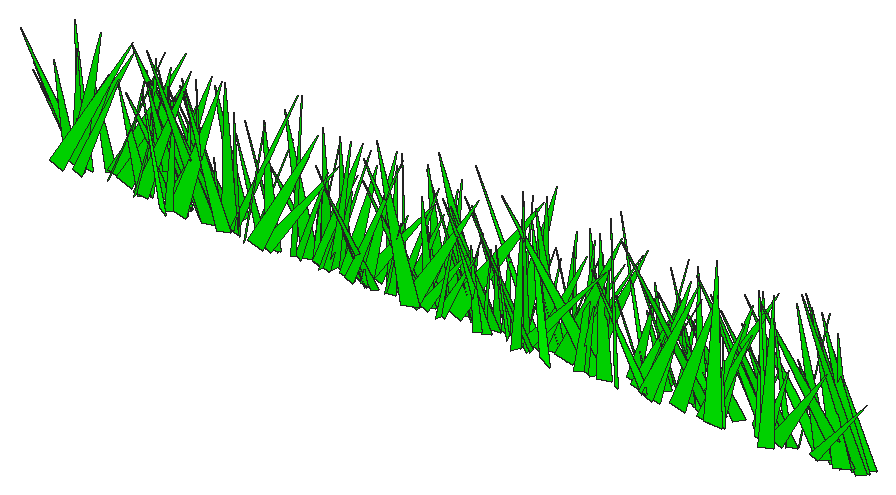
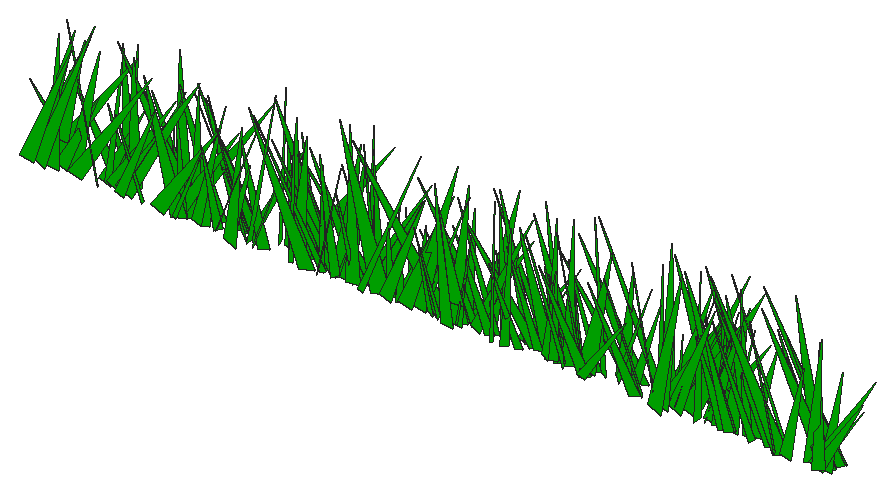
# SketchUp Ruby script. Lengths in inches.
U = 1.inch
M = Sketchup.active_model
def pt(a) = Geom::Point3d.new(a.map { |v| v * U })
def face(e, loops, mat)
  f = e.add_face(loops[0].map { |a| pt(a) })
  loops[1..].each { |l| e.add_face(l.map { |a| pt(a) }).erase! }
  f.material = f.back_material = mat if mat
  f
end
# faces: each face lists its corners as indices into pts; further lists are holes
def faces(e, pts, list, mat = nil) = list.each { |f| face(e, (f[0].is_a?(Array) ? f : [f]).map { |l| l.map { |i| pts[i] } }, mat) }
# xy, xz, yz: faces in a plane at the given z, y or x. An outline is a flat list of corners, or four numbers for a rectangle; further outlines are holes
def ring(l) = l.size == 4 ? [[l[0], l[1]], [l[2], l[1]], [l[2], l[3]], [l[0], l[3]]] : l.each_slice(2).to_a
def flat(e, list, mat, &to3) = list.each { |f| face(e, (f[0].is_a?(Array) ? f : [f]).map { |l| ring(l).map { |u, v| to3.(u, v) } }, mat) }
def xy(e, z, list, mat = nil) = flat(e, list, mat) { |x, y| [x, y, z] }
def xz(e, y, list, mat = nil) = flat(e, list, mat) { |x, z| [x, y, z] }
def yz(e, x, list, mat = nil) = flat(e, list, mat) { |y, z| [x, y, z] }
def lines(e, pts, list) = list.each { |a, b| e.add_line(pt(pts[a]), pt(pts[b])) }
# prism: a flat outline (further loops are holes) pulled along v
def prism(e, loops, v, mat = nil)
  f = face(e, loops, mat); d = Geom::Vector3d.new(v.map { |x| x * U })
  f.pushpull(f.normal.samedirection?(d) ? d.length : -d.length)
end
def box(e, o, s, mat = nil) = prism(e, [[o, [o[0] + s[0], o[1], o[2]], [o[0] + s[0], o[1] + s[1], o[2]], [o[0], o[1] + s[1], o[2]]]], [0, 0, s[2]], mat)
def at(x, y, z, deg = 0) = Geom::Transformation.translation(pt([x, y, z])) * Geom::Transformation.rotation(ORIGIN, Z_AXIS, deg.degrees)
def axes(o, x, y, z) = Geom::Transformation.new([*x, 0, *y, 0, *z, 0, *pt(o).to_a, 1])
def part(name) = M.definitions.add(name)
# library, detail: a bought-in or finely detailed component or shape, given as its bounding box
def library(name, o, s) = part(name).tap { |d| box(d.entities, o, s) }
def detail(e, o, s) = box(e.add_group.entities, o, s)
def put(e, d, t, mat = nil) = e.add_instance(d, t).tap { |i| i.material = mat if mat }
def group(e, t, mat = nil) = e.add_group.tap { |g| g.transformation = t; g.material = mat if mat }.entities
root = M.entities
M.materials.add("[0065_Lime]").color = [0, 255, 0]
c1 = part("fur_instance\#9")
p = [[0.8125,0,1.79],[0.67,-0.02,1.48],[0,-0.11,0],[0,0.11,0]]
faces(c1.entities,p,[[0,1,2,3]])
put(root,c1,axes([44.13,30.08,1.48],[-0.34451,1.18305,1.71198],[-8.4647,0.01946,-1.57758],[-1.91364,-0.29905,6.67002]),"[0065_Lime]")
put(root,c1,axes([64.73,30.03,1.48],[-8.65936,0.15726,2.6065],[-0.41279,-1.27348,1.6673],[3.36902,0.24818,6.90374]),"[0065_Lime]")
put(root,c1,axes([19.73,29.78,1.48],[-6.79777,0.33019,0.23005],[-1.91703,-0.83902,2.87402],[1.38808,0.4583,5.09585]),"[0065_Lime]")
put(root,c1,axes([61.13,30.51,1.48],[-1.56517,-0.52919,0.70817],[3.60677,-0.24741,-0.92094],[1.39004,0.0461,3.18697]),"[0065_Lime]")
put(root,c1,axes([37.86,30.3,1.48],[6.89513,0.62378,0.88009],[-4.56524,0.95182,1.05921],[-0.18718,-0.23644,6.58578]),"[0065_Lime]")
put(root,c1,axes([28.67,30.09,1.48],[2.67792,1.06969,0.54376],[-7.35877,0.33413,1.95261],[2.06045,-0.19692,6.26692]),"[0065_Lime]")
put(root,c1,axes([27.64,30.03,1.48],[6.77204,0.25909,1.43448],[-1.29307,0.95444,-1.73753],[-2.19947,0.23661,5.43816]),"[0065_Lime]")
put(root,c1,axes([23.75,30.5,1.48],[-4.80947,-1.05963,1.10538],[7.5765,-0.62399,1.76726],[-1.14397,0.32223,7.05731]),"[0065_Lime]")
put(root,c1,axes([35.81,30.94,1.48],[8.03661,-0.60589,0.58515],[3.78397,1.07013,2.74405],[-2.1888,-0.37461,6.89237]),"[0065_Lime]")
put(root,c1,axes([40.35,30.43,1.48],[-3.26499,-0.57396,0.2062],[3.89656,-0.42206,1.45586],[-1.25098,0.18336,3.99655]),"[0065_Lime]")
put(root,c1,axes([25.375,30.28,1.48],[-3.73808,0.8583,1.17661],[-6.24758,-0.48583,-1.25721],[-0.60768,-0.28494,5.6877]),"[0065_Lime]")
put(root,c1,axes([55.02,30.58,1.48],[6.37533,0.59024,0.34586],[-3.76996,0.74716,3.2521],[1.90062,-0.49786,5.29057]),"[0065_Lime]")
put(root,c1,axes([20.79,30.23,1.48],[1.96099,1.13179,1.67503],[-8.18605,0.21101,1.56321],[1.45013,-0.33931,6.55925]),"[0065_Lime]")
put(root,c1,axes([51.59,30.32,1.48],[-2.70186,0.56478,0.6732],[-4.07264,-0.35198,-0.91983],[-0.50314,-0.18378,3.83046]),"[0065_Lime]")
put(root,c1,axes([50.8,30.09,1.48],[1.71957,0.6575,0.14942],[-4.46507,0.23851,-1.16943],[-1.41103,0.04653,3.88264]),"[0065_Lime]")
put(root,c1,axes([10.625,30.42,1.48],[4.77923,0.59539,1.05401],[-4.42683,0.63025,1.35125],[0.18826,-0.29486,5.0165]),"[0065_Lime]")
put(root,c1,axes([26.14,31,1.48],[-6.87879,-0.59759,1.37199],[3.00669,-0.91307,-3.35245],[3.44834,-0.39596,5.65995]),"[0065_Lime]")
put(root,c1,axes([57.91,29.69,1.48],[-7.72011,0.59784,0.02346],[-3.67685,-0.9417,3.57075],[2.1407,0.53855,6.21771]),"[0065_Lime]")
put(root,c1,axes([41.29,30.625,1.48],[4.47026,-0.15578,0.63905],[0.86683,0.61928,1.04659],[-1.04636,-0.1525,3.59716]),"[0065_Lime]")
put(root,c1,axes([74.3,30.08,1.48],[-4.74053,1.09169,1.40979],[-7.68856,-0.70137,1.09365],[2.06121,-0.10544,7.32178]),"[0065_Lime]")
put(root,c1,axes([67.42,30.36,1.48],[4.40693,0.87518,1.12364],[-6.31769,0.56591,1.62427],[0.88649,-0.31764,5.98975]),"[0065_Lime]")
put(root,c1,axes([25.55,30.87,1.48],[-4.30465,-1.10927,0.88323],[7.70318,-0.62366,-1.40631],[2.03906,0.01431,7.17736]),"[0065_Lime]")
put(root,c1,axes([75.2,30.26,1.48],[4.33628,-0.09148,1.98024],[1.34894,0.65933,-0.93377],[-2.12858,0.23148,3.44231]),"[0065_Lime]")
put(root,c1,axes([29.49,30.375,1.48],[4.49046,0.77304,0.26708],[-5.1346,0.56521,2.2997],[2.0021,-0.28427,5.2988]),"[0065_Lime]")
put(root,c1,axes([79.83,29.84,1.48],[4.58449,1.13159,0.00259],[-7.75181,0.62024,-2.04082],[-2.18191,0.17405,7.25599]),"[0065_Lime]")
put(root,c1,axes([67.13,30.64,1.48],[-5.96088,0.35256,0.70042],[-2.64891,-0.77525,-1.83939],[-0.14148,-0.33943,4.92862]),"[0065_Lime]")
put(root,c1,axes([73.29,30.2,1.48],[2.25117,0.87167,0.12764],[-6.11845,0.30789,0.94051],[1.03451,-0.07585,5.2848]),"[0065_Lime]")
put(root,c1,axes([47.01,30.05,1.48],[4.77095,0.45802,0.17826],[-2.82349,0.60553,-2.1355],[-1.64327,0.28935,4.18681]),"[0065_Lime]")
put(root,c1,axes([46.88,30.42,1.48],[1.96891,0.5542,0.49801],[-3.85034,0.23848,1.17904],[1.05107,-0.16454,3.38624]),"[0065_Lime]")
put(root,c1,axes([55.0625,30.29,1.48],[6.20833,0.15851,0.76948],[-0.91301,0.86649,-1.1072],[-1.1549,0.16709,5.01178]),"[0065_Lime]")
put(root,c1,axes([79.29,30.27,1.48],[-7.72002,0.27436,2.22415],[-1.46785,-1.14148,1.34731],[3.0223,0.14643,6.33562]),"[0065_Lime]")
put(root,c1,axes([8.57,30.37,1.48],[6.31951,0.94895,0.38373],[-6.64339,0.85188,1.79638],[1.30162,-0.25931,7.30558]),"[0065_Lime]")
put(root,c1,axes([50.92,30.75,1.48],[4.66383,-0.24715,0.914],[1.45163,0.66185,1.09606],[-1.49965,-0.12797,3.90347]),"[0065_Lime]")
put(root,c1,axes([20.01,30.15,1.48],[4.9666,0.63068,0.82979],[-4.00726,0.69624,-1.86276],[-2.26436,0.15119,5.11659]),"[0065_Lime]")
put(root,c1,axes([45.54,30.77,1.48],[3.44033,-0.73712,1.23832],[5.16094,0.52147,0.91463],[-1.78892,0.08682,5.02012]),"[0065_Lime]")
put(root,c1,axes([16.79,30.68,1.48],[6.10882,-0.83592,0.8865],[6.04609,0.83886,-1.06071],[0.14556,0.23793,6.85422]),"[0065_Lime]")
put(root,c1,axes([32.51,30.69,1.48],[4.99618,0.36132,1.26543],[-2.96362,0.66273,1.40103],[-0.49883,-0.31852,4.35057]),"[0065_Lime]")
put(root,c1,axes([39.4375,30.48,1.48],[6.62538,-0.58044,2.05985],[4.64151,0.93329,-1.0652],[-1.39009,0.34976,6.26085]),"[0065_Lime]")
put(root,c1,axes([62.41,30.6,1.48],[-6.33645,0.9512,0.7679],[-6.40253,-0.76277,-3.29464],[-2.39198,-0.47808,6.78446]),"[0065_Lime]")
put(root,c1,axes([70.49,30.48,1.48],[1.48206,0.96371,1.77197],[-7.03462,0.12823,1.556],[1.5151,-0.34732,5.49117]),"[0065_Lime]")
put(root,c1,axes([73.43,30.62,1.48],[0.03926,-0.79438,1.85545],[5.57297,-0.12523,-1.87468],[2.47072,0.2951,4.19905]),"[0065_Lime]")
put(root,c1,axes([54.85,29.86,1.48],[6.6919,0.91235,0.39414],[-5.64636,0.86183,-3.41967],[-3.24188,0.38224,6.76961]),"[0065_Lime]")
put(root,c1,axes([53.22,30.93,1.48],[-5.33765,-0.0585,1.68343],[-0.58614,-0.71856,-2.06642],[2.02805,-0.36165,3.83342]),"[0065_Lime]")
put(root,c1,axes([55.17,30.85,1.48],[7.44197,0.33682,3.48445],[-3.54431,1.12505,1.36438],[-3.39614,-0.43606,6.21157]),"[0065_Lime]")
put(root,c1,axes([39.33,30.36,1.48],[-6.258,-0.06196,0.08284],[0.4498,-0.82981,1.68502],[-0.04972,0.29136,4.81674]),"[0065_Lime]")
put(root,c1,axes([43.83,30.37,1.48],[2.93679,1.03445,0.45779],[-7.01385,0.3643,2.1857],[2.30591,-0.20936,6.06519]),"[0065_Lime]")
put(root,c1,axes([44.99,30.75,1.48],[-2.764,-0.83685,0.50313],[5.63527,-0.33124,2.02156],[-2.02329,0.22064,4.94315]),"[0065_Lime]")
put(root,c1,axes([19.54,30.7,1.48],[2.11424,-0.60397,0.5987],[4.26926,0.26326,-1.07586],[0.88853,0.17219,3.74479]),"[0065_Lime]")
put(root,c1,axes([10.47,30.74,1.48],[4.9323,0.07226,0.38753],[-0.61627,0.6737,0.98048],[-0.33408,-0.17598,3.91277]),"[0065_Lime]")
put(root,c1,axes([45.11,30.5,1.48],[1.61128,0.64633,0.39163],[-4.24285,0.17808,1.70173],[1.8403,-0.15533,3.5805]),"[0065_Lime]")
put(root,c1,axes([16.42,30.35,1.48],[5.70875,0.27855,0.71591],[-1.6723,0.78704,-1.43816],[-1.38113,0.19838,4.70047]),"[0065_Lime]")
put(root,c1,axes([8.36,30.5625,1.48],[5.86152,-0.41679,0.56137],[3.03624,0.7836,-1.48096],[0.23491,0.2716,5.13419]),"[0065_Lime]")
put(root,c1,axes([79.91,30.92,1.48],[1.05734,-0.86071,0.08127],[5.5355,0.12813,-2.17864],[2.62437,0.07651,4.56261]),"[0065_Lime]")
put(root,c1,axes([55.96,30.4,1.48],[-7.62078,-0.34843,0.45683],[2.49237,-0.9746,2.60079],[-0.50201,0.45068,5.97743]),"[0065_Lime]")
put(root,c1,axes([62.59,31.22,1.48],[-5.45062,-0.70546,0.87197],[4.01856,-0.72305,-2.98167],[3.19451,-0.29412,5.2386]),"[0065_Lime]")
put(root,c1,axes([25.02,30.79,1.48],[-3.37114,-0.68743,0.25691],[4.73176,-0.44219,1.43322],[-1.28176,0.17559,4.61519]),"[0065_Lime]")
put(root,c1,axes([20.11,31.16,1.48],[1.9608,-1.03944,0.05335],[7.06022,0.2658,1.84469],[-2.20827,-0.07315,5.94518]),"[0065_Lime]")
put(root,c1,axes([67,30.93,1.48],[7.46045,-0.02634,0.01423],[0.17757,1.01684,1.47697],[-0.06257,-0.25501,5.88792]),"[0065_Lime]")
put(root,c1,axes([35.02,30.3125,1.48],[4.95164,0.33086,0.06413],[-2.09705,0.63075,-1.91146],[-1.07357,0.29394,4.02952]),"[0065_Lime]")
put(root,c1,axes([21.18,30.44,1.48],[-4.20396,0.56015,1.05282],[-3.63846,-0.61562,1.36277],[2.08029,0.05524,4.51112]),"[0065_Lime]")
put(root,c1,axes([63.3,30.37,1.48],[3.53617,1.02426,1.11587],[-7.09395,0.5294,-1.409],[-2.16561,-0.06167,6.43759]),"[0065_Lime]")
put(root,c1,axes([79.1,30.66,1.48],[-0.61437,0.59604,1.22758],[-4.24315,-0.14821,1.00633],[1.5052,-0.17452,3.33789]),"[0065_Lime]")
put(root,c1,axes([73.74,30.77,1.48],[-7.08166,-0.81662,0.17362],[5.52934,-0.93086,2.50861],[-1.80162,0.35301,7.01671]),"[0065_Lime]")
put(root,c1,axes([38.75,30.74,1.48],[4.21896,0.77814,0.50808],[-5.12819,0.49902,2.56524],[2.18119,-0.33188,5.04839]),"[0065_Lime]")
put(root,c1,axes([60.83,30.25,1.48],[5.77702,0.78384,0.4571],[-5.17205,0.78886,-2.08011],[-2.16388,0.20714,6.19215]),"[0065_Lime]")
put(root,c1,axes([58.75,30.97,1.48],[3.38346,-1.14343,0.9649],[8.00166,0.41622,-2.0368],[1.8963,0.28388,6.87288]),"[0065_Lime]")
put(root,c1,axes([9.89,31.22,1.48],[-2.76887,-1.21381,1.08117],[8.19055,-0.42874,-2.25062],[3.04935,0.04944,7.02687]),"[0065_Lime]")
put(root,c1,axes([24.23,31.12,1.48],[4.01821,-0.27298,0.79897],[1.21611,0.52182,1.92753],[-1.80549,-0.25605,3.07644]),"[0065_Lime]")
put(root,c1,axes([51.7,31.08,1.48],[-3.47012,-0.89722,0.02546],[6.3041,-0.48062,0.95274],[-1.01439,0.08241,5.83391]),"[0065_Lime]")
put(root,c1,axes([67.98,30.36,1.48],[-0.54683,1.10854,0.02669],[-7.62502,-0.07545,1.64848],[2.02398,0.01525,6.21759]),"[0065_Lime]")
put(root,c1,axes([81.49,31.04,1.48],[-2.34472,-0.69785,0.00894],[4.84361,-0.32096,0.99094],[-1.09707,0.07445,4.35595]),"[0065_Lime]")
put(root,c1,axes([34.79,30.67,1.48],[-0.02453,1.07017,1.82422],[-7.63781,-0.08919,1.68541],[2.16693,-0.30227,5.96124]),"[0065_Lime]")
put(root,c1,axes([30.25,30.4,1.48],[1.12595,1.02406,0.02745],[-7.14073,0.15598,-1.19488],[-1.45681,0.02692,5.87806]),"[0065_Lime]")
put(root,c1,axes([41.82,30.57,1.48],[4.58876,0.78387,1.2447],[-5.43643,0.67819,-1.05087],[-1.97632,-0.0455,5.78077]),"[0065_Lime]")
put(root,c1,axes([56.26,30.8125,1.48],[3.26519,0.80916,1.18068],[-5.80446,0.38567,1.76398],[1.25481,-0.32151,5.08744]),"[0065_Lime]")
put(root,c1,axes([81.05,31.17,1.48],[6.31811,-0.3726,2.29669],[1.81831,0.95557,1.88518],[-3.42013,-0.1803,5.245]),"[0065_Lime]")
put(root,c1,axes([21.06,30.85,1.48],[-2.16414,0.7747,1.25751],[-5.23696,-0.17391,-2.37307],[-2.31508,-0.33079,4.19263]),"[0065_Lime]")
put(root,c1,axes([24.67,30.82,1.48],[-4.78974,-0.70249,1.35936],[5.20184,-0.5786,2.10767],[-0.85263,0.41637,5.2224]),"[0065_Lime]")
put(root,c1,axes([83.74,30.93,1.48],[3.13394,-0.51874,0.22908],[3.37163,0.37845,-1.80201],[1.52966,0.22863,3.50261]),"[0065_Lime]")
put(root,c1,axes([37.44,30.6,1.48],[0.27303,0.99371,0.50679],[-6.98624,0.02204,1.04194],[1.26131,-0.09301,5.6615]),"[0065_Lime]")
put(root,c1,axes([34.89,31.43,1.48],[-5.54195,-0.92621,0.82807],[6.12637,-0.78045,-2.12354],[2.63644,-0.13338,6.67517]),"[0065_Lime]")
put(root,c1,axes([32.02,30.66,1.48],[-7.66197,-0.27152,3.61915],[3.16093,-1.16605,1.49624],[3.67952,0.43631,6.2509]),"[0065_Lime]")
put(root,c1,axes([44.3,31.3,1.48],[-7.1206,0.3926,1.63931],[-3.42947,-0.86949,-2.87834],[0.32662,-0.57038,5.5161]),"[0065_Lime]")
put(root,c1,axes([25.9,30.84,1.48],[9.19632,-0.27126,0.84978],[2.08385,1.27761,-1.25483],[-0.68968,0.24321,7.53973]),"[0065_Lime]")
put(root,c1,axes([17.05,30.78,1.48],[0.28843,0.82416,1.15249],[-5.76326,0.09666,-1.36183],[-1.78688,-0.17871,4.57835]),"[0065_Lime]")
put(root,c1,axes([38.28,30.91,1.48],[2.96676,0.61035,0.96182],[-4.48697,0.38487,0.97325],[0.36324,-0.2308,4.16645]),"[0065_Lime]")
put(root,c1,axes([28.93,30.74,1.48],[2.6731,0.66495,1.57301],[-4.18891,0.46068,-1.8158],[-2.93023,-0.05197,4.03076]),"[0065_Lime]")
put(root,c1,axes([24.37,31.28,1.48],[-7.38884,-0.17704,0.81253],[0.97677,-1.0186,-1.56024],[1.27719,-0.24524,5.89391]),"[0065_Lime]")
put(root,c1,axes([44.65,30.94,1.48],[4.65614,-0.28083,0.65176],[2.13954,0.63358,-0.96525],[-0.24196,0.19831,4.00688]),"[0065_Lime]")
put(root,c1,axes([30.59,30.64,1.48],[-6.85125,-0.10613,1.12079],[1.32002,-0.85859,2.61458],[0.85238,0.4766,4.9597]),"[0065_Lime]")
put(root,c1,axes([34.17,30.74,1.48],[-2.94845,0.40649,0.32779],[-2.55851,-0.39827,1.32291],[1.40883,0.12745,3.08848]),"[0065_Lime]")
put(root,c1,axes([42.36,31.1,1.48],[6.1199,0.46646,1.25038],[-3.61354,0.83643,1.24592],[-0.5702,-0.29422,5.52443]),"[0065_Lime]")
put(root,c1,axes([86.88,31.12,1.48],[-4.12975,-1.07405,1.04713],[7.15683,-0.44965,3.22052],[-2.97669,0.40901,6.29031]),"[0065_Lime]")
put(root,c1,axes([13.12,31.32,1.48],[9.12899,-0.0554,0.62058],[0.2297,1.26046,1.53488],[-0.8275,-0.2613,7.27235]),"[0065_Lime]")
put(root,c1,axes([36.53,31.47,1.48],[-4.4726,-0.95185,0.9019],[6.54021,-0.64741,-1.43618],[2.08342,-0.01107,6.44459]),"[0065_Lime]")
put(root,c1,axes([78.88,30.51,1.48],[-6.08081,0.9053,0.32826],[-6.02582,-0.824,2.29337],[2.31511,0.23312,6.83143]),"[0065_Lime]")
put(root,c1,axes([23.14,31.22,1.48],[0.19669,-1.17509,2.75798],[7.93251,0.24969,3.19052],[-4.30161,0.40672,6.00967]),"[0065_Lime]")
put(root,c1,axes([35.77,31.46,1.48],[-1.59698,-0.7417,0.12759],[4.95284,-0.21837,-1.51964],[1.83164,-0.0562,4.22043]),"[0065_Lime]")
put(root,c1,axes([18.72,31.52,1.48],[1.39332,-0.98147,0.23166],[6.8751,0.19978,1.00274],[-1.26478,0.00474,5.70592]),"[0065_Lime]")
put(root,c1,axes([65.93,30.98,1.48],[2.17124,0.69862,0.42174],[-4.89291,0.28077,1.08165],[1.023,-0.13985,4.2783]),"[0065_Lime]")
put(root,c1,axes([73.3,31.47,1.48],[4.48042,-0.50548,0.43047],[3.35712,0.62043,1.29372],[-1.39651,-0.13027,4.49111]),"[0065_Lime]")
put(root,c1,axes([78.88,31.23,1.48],[-6.31778,0.51578,0.77321],[-3.78287,-0.83978,-1.67965],[-0.25767,-0.31737,5.70105]),"[0065_Lime]")
put(root,c1,axes([80.44,31.24,1.48],[-2.66226,-0.86902,1.05673],[5.91511,-0.27297,2.33785],[-2.22407,0.31426,4.95277]),"[0065_Lime]")
put(root,c1,axes([21.71,31.82,1.48],[-7.39918,-0.69801,1.4198],[3.67901,-0.98805,-3.59127],[3.76651,-0.40612,6.297]),"[0065_Lime]")
put(root,c1,axes([16.99,31.47,1.48],[7.09272,-0.46853,1.73214],[2.97386,1.0365,1.33786],[-2.60934,-0.09227,6.23306]),"[0065_Lime]")
put(root,c1,axes([72.32,31.11,1.48],[5.4685,-0.97873,1.76259],[7.06858,0.61705,-3.02887],[1.80115,0.54994,6.53532]),"[0065_Lime]")
put(root,c1,axes([88.39,31.05,1.48],[-7.38794,-0.72693,1.68669],[5.57161,-0.95117,2.41034],[-0.13975,0.50783,6.92899]),"[0065_Lime]")
put(root,c1,axes([79.35,31.34,1.48],[-2.65206,-1.11272,1.30021],[7.52645,-0.25445,2.86065],[-2.93492,0.35297,6.16111]),"[0065_Lime]")
put(root,c1,axes([54.45,31.33,1.48],[-3.74352,-0.72471,0.61157],[5.12081,-0.4872,1.39333],[-0.97047,0.22473,4.99299]),"[0065_Lime]")
put(root,c1,axes([19.96,31.57,1.48],[-4.65073,-0.7053,0.80494],[4.80467,-0.66671,-1.20795],[1.7572,-0.04373,5.43329]),"[0065_Lime]")
put(root,c1,axes([74.08,31.32,1.48],[-1.37559,-0.85863,1.37948],[5.69675,-0.06019,2.50319],[-2.78596,0.30088,4.43741]),"[0065_Lime]")
put(root,c1,axes([57.77,31.42,1.48],[1.29418,-1.03641,1.94954],[7.57285,0.24251,0.9938],[-1.67218,0.29612,6.00948]),"[0065_Lime]")
put(root,c1,axes([65.87,31.27,1.48],[3.96145,-0.59181,0.80933],[4.28645,0.51053,-1.37254],[0.59515,0.26225,4.49838]),"[0065_Lime]")
put(root,c1,axes([69.89,31.625,1.48],[-6.84154,-0.18766,0.54844],[1.10373,-0.93253,-1.58239],[1.00991,-0.25212,5.44475]),"[0065_Lime]")
put(root,c1,axes([14.53,31.42,1.48],[0.52255,-0.98343,1.97503],[6.73947,-0.07887,-2.49575],[3.07507,0.33997,5.13418]),"[0065_Lime]")
put(root,c1,axes([57.79,31.61,1.48],[-4.37894,-0.24579,0.25921],[1.54269,-0.58443,-1.32615],[0.88383,-0.19765,3.59898]),"[0065_Lime]")
put(root,c1,axes([16.74,31.2,1.48],[-0.17243,1.01818,1.85751],[-7.46698,-0.0819,1.04571],[1.40096,-0.3112,5.80214]),"[0065_Lime]")
put(root,c1,axes([42.76,31.36,1.48],[2.93102,0.63234,1.28937],[-4.71074,0.3421,1.46325],[0.75651,-0.3197,4.11603]),"[0065_Lime]")
put(root,c1,axes([9.6,31.41,1.48],[2.45025,0.6353,1.67572],[-4.88555,0.2494,1.55826],[0.90345,-0.37436,3.88183]),"[0065_Lime]")
put(root,c1,axes([70.83,31.6875,1.48],[-3.03581,-0.57435,0.05824],[3.90225,-0.41088,-1.19279],[1.21821,-0.11514,3.96594]),"[0065_Lime]")
put(root,c1,axes([50.01,31.43,1.48],[-3.66849,1.04125,2.72934],[-8.1151,-0.43288,-1.68299],[-0.55978,-0.54832,6.51168]),"[0065_Lime]")
put(root,c1,axes([65.07,31.66,1.48],[-0.76658,-0.82654,0.56432],[5.61439,-0.13271,-1.46741],[1.88649,0.05911,4.59647]),"[0065_Lime]")
put(root,c1,axes([58.67,31.11,1.48],[6.90967,-0.254,0.67591],[1.98945,0.88454,-2.31761],[-0.01117,0.41705,5.32726]),"[0065_Lime]")
put(root,c1,axes([85.66,31.22,1.48],[-0.52226,0.7386,0.75982],[-4.94057,-0.0169,-1.69652],[-2.02281,-0.14943,3.94745]),"[0065_Lime]")
put(root,c1,axes([88.18,31.26,1.48],[-0.7267,1.1109,2.0205],[-8.0479,-0.01108,-1.71103],[-1.97557,-0.3635,6.22698]),"[0065_Lime]")
put(root,c1,axes([56.24,31.65,1.48],[-5.00755,-0.9574,2.00572],[6.74141,-0.76999,-1.18005],[2.6563,0.1493,6.77594]),"[0065_Lime]")
put(root,c1,axes([8.95,31.75,1.48],[1.13429,-0.83246,0.19665],[5.81159,0.16295,0.93549],[-1.1751,0.00234,4.8164]),"[0065_Lime]")
put(root,c1,axes([46.13,31.6875,1.48],[3.35135,-0.99937,1.51948],[7.03532,0.51969,1.18677],[-2.139,0.1435,6.28408]),"[0065_Lime]")
put(root,c1,axes([51.54,31.68,1.48],[-2.03029,-0.50556,0.08752],[3.43677,-0.27743,-0.9516],[1.06992,-0.06819,3.22279]),"[0065_Lime]")
put(root,c1,axes([86.53,30.875,1.48],[1.50451,1.24562,0.17558],[-8.40447,0.21013,-2.30329],[-2.8268,0.03822,6.94146]),"[0065_Lime]")
put(root,c1,axes([49.41,31.32,1.48],[-7.18343,-0.37485,1.05181],[2.90341,-0.98579,1.34735],[0.59874,0.28304,6.08562]),"[0065_Lime]")
put(root,c1,axes([57.96,31.25,1.48],[6.38859,0.05573,0.59544],[-0.2448,0.88654,-1.04236],[-0.79574,0.17465,5.10116]),"[0065_Lime]")
put(root,c1,axes([47.41,31.2,1.48],[3.40621,1.21547,0.59163],[-7.99189,0.39626,3.16396],[3.38825,-0.28725,6.8681]),"[0065_Lime]")
put(root,c1,axes([33.41,31.02,1.48],[1.33291,1.13033,0.60445],[-7.71462,0.2095,-1.87221],[-2.39665,-0.04573,6.36264]),"[0065_Lime]")
put(root,c1,axes([50.96,31.78,1.48],[0.02235,-0.94554,0.30429],[6.44057,0.01847,1.61066],[-1.98436,0.04931,5.23109]),"[0065_Lime]")
put(root,c1,axes([33.27,31.76,1.48],[7.41782,-0.13926,1.17124],[0.54514,1.02244,1.78935],[-1.66084,-0.2864,5.81844]),"[0065_Lime]")
put(root,c1,axes([45.77,31.63,1.48],[-4.7989,0.07802,1.51802],[-1.11652,-0.6817,-1.16126],[1.59516,-0.24243,3.75402]),"[0065_Lime]")
put(root,c1,axes([72.5625,30.9,1.48],[-6.69958,0.7682,0.43825],[-4.99148,-0.90113,2.44316],[2.29408,0.28275,6.59568]),"[0065_Lime]")
put(root,c1,axes([20.83,31.3125,1.48],[-2.67199,0.79999,0.78385],[-5.74037,-0.35192,-0.91153],[-0.62342,-0.1883,5.03368]),"[0065_Lime]")
put(root,c1,axes([18.9,31.57,1.48],[-0.39707,-1.07013,2.43728],[7.75544,-0.18381,-1.86838],[2.61332,0.38289,5.91502]),"[0065_Lime]")
put(root,c1,axes([81.58,31.86,1.48],[8.61496,-0.02408,1.61525],[-0.44714,1.18302,2.16892],[-1.94235,-0.37915,6.66487]),"[0065_Lime]")
put(root,c1,axes([54.14,31.21,1.48],[7.78645,0.00536,2.58731],[0.90729,1.129,-1.88493],[-3.0489,0.34965,6.0467]),"[0065_Lime]")
put(root,c1,axes([86.11,31.85,1.48],[4.74162,-0.82711,1.23492],[5.64643,0.69949,1.35443],[-2.25163,0.01234,5.99709]),"[0065_Lime]")
put(root,c1,axes([40.87,31.9375,1.48],[-4.70089,-0.69903,0.72009],[4.58609,-0.66159,-1.71198],[2.12104,-0.11878,5.29756]),"[0065_Lime]")
put(root,c1,axes([25.55,31.5625,1.48],[-5.11531,-0.58292,0.33608],[4.04956,-0.67294,1.66959],[-0.99049,0.2592,5.09034]),"[0065_Lime]")
put(root,c1,axes([33.59,31.26,1.48],[4.48183,0.17345,1.2207],[-0.43428,0.60613,-1.83102],[-1.89399,0.27146,3.30843]),"[0065_Lime]")
put(root,c1,axes([9.43,32.12,1.48],[-3.94012,-0.92854,0.03739],[6.23516,-0.52488,-2.05179],[2.18882,-0.17629,5.91211]),"[0065_Lime]")
put(root,c1,axes([37.27,31.39,1.48],[-4.35608,-0.30765,1.92976],[2.99848,-0.59304,1.31024],[1.19624,0.36621,3.74296]),"[0065_Lime]")
put(root,c1,axes([8.84,31.65,1.48],[2.8886,-1.04803,1.65082],[7.33954,0.27642,-2.61701],[2.42419,0.41192,5.95625]),"[0065_Lime]")
put(root,c1,axes([59.26,31.62,1.48],[7.28594,0.47401,0.17386],[-3.33788,0.99775,1.39732],[0.53253,-0.23145,6.37963]),"[0065_Lime]")
put(root,c1,axes([59.43,32.01,1.48],[-6.31669,-0.24547,1.10563],[1.06218,-0.84289,-2.25566],[1.94191,-0.33743,4.83022]),"[0065_Lime]")
put(root,c1,axes([84.5625,31.07,1.48],[3.3021,1.13593,0.67248],[-7.35859,0.4712,-2.76355],[-3.44725,0.08227,6.5433]),"[0065_Lime]")
put(root,c1,axes([59.61,31.34,1.48],[5.21765,0.45216,1.60903],[-2.62793,0.77503,-1.65979],[-2.71317,0.11886,4.70196]),"[0065_Lime]")
put(root,c1,axes([62.12,31.2,1.48],[1.45379,1.11657,0.33703],[-7.8012,0.21167,-1.23306],[-1.56636,-0.01787,6.45402]),"[0065_Lime]")
put(root,c1,axes([77.01,31.85,1.48],[4.40491,0.16716,0.77862],[-1.49737,0.55331,1.62428],[-0.29895,-0.30832,3.33707]),"[0065_Lime]")
put(root,c1,axes([73.37,31.9,1.48],[0.30414,-1.02536,1.10172],[7.14044,-0.01151,-1.66309],[2.02349,0.19472,5.70307]),"[0065_Lime]")
put(root,c1,axes([71.85,31.61,1.48],[-5.50256,-0.60636,1.7261],[4.73414,-0.76258,1.0088],[0.84358,0.3244,5.59783]),"[0065_Lime]")
put(root,c1,axes([52.63,31.38,1.48],[-3.03044,0.50656,0.34814],[-3.38287,-0.42247,1.11517],[1.31724,0.08043,3.66485]),"[0065_Lime]")
put(root,c1,axes([21.22,31.43,1.48],[-7.29423,-0.00471,1.06323],[0.37598,-1.00456,1.55747],[1.25233,0.27415,5.72522]),"[0065_Lime]")
put(root,c1,axes([27.49,31.48,1.48],[6.27759,0.0987,0.63897],[-0.50068,0.86608,-1.22808],[-0.92721,0.20054,4.98922]),"[0065_Lime]")
put(root,c1,axes([67.55,31.05,1.48],[8.25078,0.54059,0.57891],[-3.13796,1.05378,-3.38295],[-2.3367,0.49368,6.58708]),"[0065_Lime]")
put(root,c1,axes([66,31.91,1.48],[-4.76929,-0.07793,0.52998],[0.34987,-0.65078,-1.12321],[0.78079,-0.18438,3.74054]),"[0065_Lime]")
put(root,c1,axes([83.9375,31.63,1.48],[-5.81397,0.81729,0.09522],[-5.55244,-0.77265,-2.0866],[-1.73581,-0.26591,6.3556]),"[0065_Lime]")
put(root,c1,axes([56.3,31.27,1.48],[-5.14256,0.39956,1.40476],[-1.46436,-0.67302,2.86772],[2.98724,0.35793,3.82408]),"[0065_Lime]")
put(root,c1,axes([19.15,31.78,1.48],[1.32281,-0.61534,1.27181],[4.55604,0.12587,-1.09468],[0.92934,0.2588,3.55631]),"[0065_Lime]")
put(root,c1,axes([68.24,32.02,1.48],[2.36285,-0.5655,0.72455],[3.59854,0.35337,1.4774],[-2.01,-0.03213,3.49675]),"[0065_Lime]")
put(root,c1,axes([24.875,32.0625,1.48],[3.26689,-0.49068,0.65678],[3.08636,0.46319,1.4383],[-1.82205,-0.09517,3.61392]),"[0065_Lime]")
put(root,c1,axes([53.48,31.58,1.48],[-0.42066,1.25732,2.14574],[-9.03671,-0.14701,1.71431],[2.31502,-0.34538,7.08174]),"[0065_Lime]")
put(root,c1,axes([62.2,31.96,1.48],[5.50173,0.23721,2.52605],[-2.46488,0.83611,0.92105],[-2.53342,-0.29835,4.5896]),"[0065_Lime]")
put(root,c1,axes([39.6,31.7,1.48],[1.79791,0.57193,0.56257],[-4.05181,0.22411,0.93321],[0.79204,-0.15181,3.49696]),"[0065_Lime]")
put(root,c1,axes([66.6875,31.51,1.48],[-8.99054,0.23905,1.68066],[-1.29453,-1.27904,1.51413],[2.3425,0.21063,7.28715]),"[0065_Lime]")
put(root,c1,axes([18.58,31.78,1.48],[3.92587,-0.56625,1.3255],[4.34011,0.52766,-0.95167],[-0.2398,0.27987,4.47616]),"[0065_Lime]")
put(root,c1,axes([52.82,31.86,1.48],[-3.46115,-0.75636,1.112],[5.52551,-0.44627,1.20769],[-0.55779,0.27255,5.06337]),"[0065_Lime]")
put(root,c1,axes([69.8,31.41,1.48],[-3.31762,0.59533,0.25097],[-3.71549,-0.43334,1.94815],[2.05912,0.17726,3.91961]),"[0065_Lime]")
put(root,c1,axes([48.55,31.57,1.48],[2.80633,0.43003,0.01815],[-2.9341,0.37926,-0.94446],[-0.87027,0.10805,3.24276]),"[0065_Lime]")
put(root,c1,axes([27.97,31.86,1.48],[1.19323,-0.7479,1.56625],[5.26781,0.04559,-1.92581],[2.07047,0.31503,3.99711]),"[0065_Lime]")
put(root,c1,axes([42.09,32.08,1.48],[-6.86894,-0.37341,2.2376],[2.19522,-1.03555,-1.33212],[3.13211,-0.09313,5.84086]),"[0065_Lime]")
put(root,c1,axes([75.55,31.9,1.48],[-1.07484,-0.85828,1.77554],[5.76558,0.01602,2.56876],[-2.97164,0.34152,4.34168]),"[0065_Lime]")
put(root,c1,axes([55.09,32.1,1.48],[-9.07347,0.15417,1.04909],[-1.38985,-1.24237,-1.83564],[0.96718,-0.33902,7.20405]),"[0065_Lime]")
put(root,c1,axes([12.65,32.16,1.48],[2.68036,-0.6741,0.73821],[4.45394,0.39719,1.45384],[-2.00003,-0.01889,4.22692]),"[0065_Lime]")
put(root,c1,axes([10.04,31.76,1.48],[-4.44766,0.76438,0.04936],[-5.21747,-0.59625,-1.65688],[-1.54024,-0.1875,5.47005]),"[0065_Lime]")
put(root,c1,axes([45.625,31.43,1.48],[-2.94392,0.9556,0.12745],[-6.46635,-0.40058,1.81859],[2.11156,0.10557,5.74686]),"[0065_Lime]")
put(root,c1,axes([88.5,31.91,1.48],[-4.42327,0.76958,1.40872],[-5.72897,-0.56882,-1.48913],[-0.41597,-0.34926,5.52933]),"[0065_Lime]")
put(root,c1,axes([79.3,31.89,1.48],[-3.63836,-0.59296,1.15803],[4.43912,-0.46211,1.29902],[-0.35771,0.2964,4.34199]),"[0065_Lime]")
put(root,c1,axes([9.55,31.86,1.48],[-4.09291,-0.33198,0.12298],[2.26755,-0.53755,1.30657],[-0.68029,0.20557,3.61521]),"[0065_Lime]")
put(root,c1,axes([73.71,32.04,1.48],[-4.73366,0.1045,0.64784],[-0.9251,-0.64903,-0.9643],[0.57582,-0.18365,3.77648]),"[0065_Lime]")
put(root,c1,axes([47.61,31.67,1.48],[5.00478,-0.01945,1.00789],[0.61574,0.66487,-1.59301],[-1.08415,0.28782,3.74802]),"[0065_Lime]")
put(root,c1,axes([60.37,32.17,1.48],[5.08956,-0.93975,0.10992],[6.58612,0.69984,-1.27738],[1.16943,0.1485,6.71565]),"[0065_Lime]")
put(root,c1,axes([35.31,31.48,1.48],[7.49226,0.10431,1.25474],[-0.01036,0.97586,-2.67747],[-1.71184,0.45062,5.50784]),"[0065_Lime]")
put(root,c1,axes([25.43,32.57,1.48],[5.93133,-0.9014,0.88146],[5.35138,0.79317,3.35433],[-3.6996,-0.29784,6.26514]),"[0065_Lime]")
put(root,c1,axes([67.75,32.58,1.48],[5.61852,-0.73317,0.08525],[4.50757,0.69269,3.0634],[-2.62989,-0.37909,5.43271]),"[0065_Lime]")
put(root,c1,axes([32.89,31.86,1.48],[1.63792,0.76095,0.99592],[-5.26457,0.1559,1.7372],[1.76332,-0.24139,4.2615]),"[0065_Lime]")
put(root,c1,axes([13.21,31.99,1.48],[6.26643,-0.91717,0.97292],[6.53867,0.81405,-2.14993],[1.13098,0.37541,7.03895]),"[0065_Lime]")
put(root,c1,axes([9.6,31.93,1.48],[-1.88891,0.64714,0.87236],[-4.41407,-0.18311,-1.77199],[-1.69584,-0.24419,3.6406]),"[0065_Lime]")
put(root,c1,axes([58,31.64,1.48],[-5.51931,0.58625,1.7056],[-3.51703,-0.82202,1.93758],[3.07137,0.1122,5.28373]),"[0065_Lime]")
put(root,c1,axes([24.14,31.625,1.48],[2.52658,0.96537,1.40653],[-6.03763,0.42837,-2.67624],[-3.70608,-0.03974,5.31879]),"[0065_Lime]")
put(root,c1,axes([16.32,31.76,1.48],[6.19612,-0.23798,1.22147],[2.12866,0.82173,-1.77956],[-0.76952,0.35685,4.9125]),"[0065_Lime]")
put(root,c1,axes([46.35,32.29,1.48],[6.05593,-0.66106,1.1075],[4.53759,0.87183,1.02095],[-1.84277,-0.02567,6.15355]),"[0065_Lime]")
put(root,c1,axes([10.62,31.49,1.48],[-5.68106,0.87786,0.09687],[-6.06169,-0.77977,1.58124],[1.51633,0.17175,6.68409]),"[0065_Lime]")
put(root,c1,axes([33.125,32.04,1.48],[-2.93413,0.46934,0.54979],[-3.22303,-0.34149,-1.61217],[-1.10685,-0.24979,3.23704]),"[0065_Lime]")
put(root,c1,axes([13.67,32.24,1.48],[6.69209,0.12062,1.44856],[-1.35303,0.92345,1.55907],[-1.44138,-0.30682,5.26192]),"[0065_Lime]")
put(root,c1,axes([87.36,31.89,1.48],[-6.2814,-0.82129,2.04556],[6.36097,-0.79873,2.17782],[-0.15144,0.51571,6.6306]),"[0065_Lime]")
